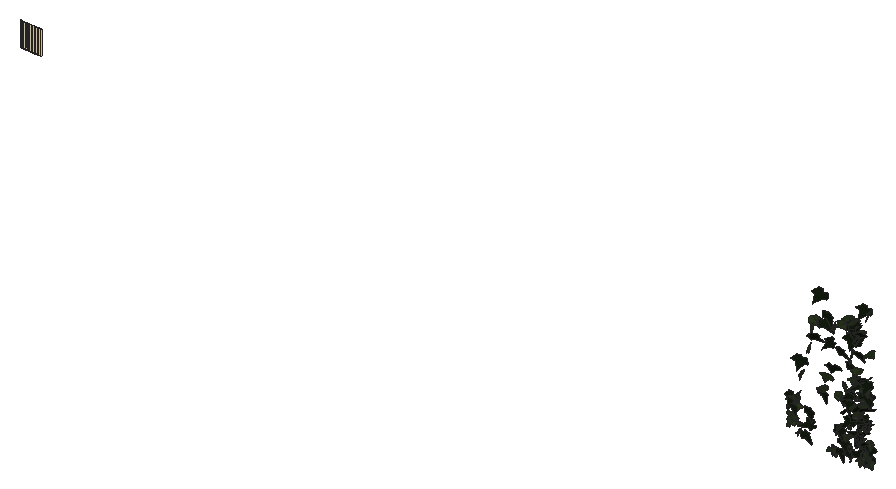
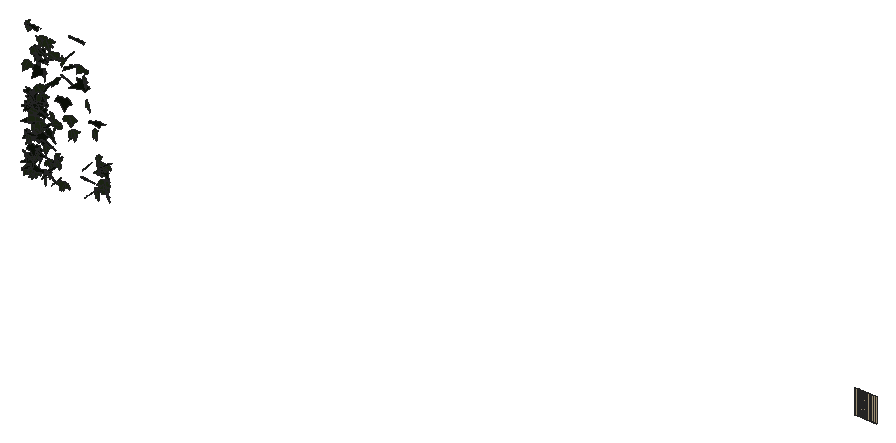
# SketchUp Ruby script. Lengths in inches.
U = 1.inch
M = Sketchup.active_model
def pt(a) = Geom::Point3d.new(a.map { |v| v * U })
def face(e, loops, mat)
  f = e.add_face(loops[0].map { |a| pt(a) })
  loops[1..].each { |l| e.add_face(l.map { |a| pt(a) }).erase! }
  f.material = f.back_material = mat if mat
  f
end
# faces: each face lists its corners as indices into pts; further lists are holes
def faces(e, pts, list, mat = nil) = list.each { |f| face(e, (f[0].is_a?(Array) ? f : [f]).map { |l| l.map { |i| pts[i] } }, mat) }
# xy, xz, yz: faces in a plane at the given z, y or x. An outline is a flat list of corners, or four numbers for a rectangle; further outlines are holes
def ring(l) = l.size == 4 ? [[l[0], l[1]], [l[2], l[1]], [l[2], l[3]], [l[0], l[3]]] : l.each_slice(2).to_a
def flat(e, list, mat, &to3) = list.each { |f| face(e, (f[0].is_a?(Array) ? f : [f]).map { |l| ring(l).map { |u, v| to3.(u, v) } }, mat) }
def xy(e, z, list, mat = nil) = flat(e, list, mat) { |x, y| [x, y, z] }
def xz(e, y, list, mat = nil) = flat(e, list, mat) { |x, z| [x, y, z] }
def yz(e, x, list, mat = nil) = flat(e, list, mat) { |y, z| [x, y, z] }
def lines(e, pts, list) = list.each { |a, b| e.add_line(pt(pts[a]), pt(pts[b])) }
# prism: a flat outline (further loops are holes) pulled along v
def prism(e, loops, v, mat = nil)
  f = face(e, loops, mat); d = Geom::Vector3d.new(v.map { |x| x * U })
  f.pushpull(f.normal.samedirection?(d) ? d.length : -d.length)
end
def box(e, o, s, mat = nil) = prism(e, [[o, [o[0] + s[0], o[1], o[2]], [o[0] + s[0], o[1] + s[1], o[2]], [o[0], o[1] + s[1], o[2]]]], [0, 0, s[2]], mat)
def at(x, y, z, deg = 0) = Geom::Transformation.translation(pt([x, y, z])) * Geom::Transformation.rotation(ORIGIN, Z_AXIS, deg.degrees)
def axes(o, x, y, z) = Geom::Transformation.new([*x, 0, *y, 0, *z, 0, *pt(o).to_a, 1])
def part(name) = M.definitions.add(name)
# library, detail: a bought-in or finely detailed component or shape, given as its bounding box
def library(name, o, s) = part(name).tap { |d| box(d.entities, o, s) }
def detail(e, o, s) = box(e.add_group.entities, o, s)
def put(e, d, t, mat = nil) = e.add_instance(d, t).tap { |i| i.material = mat if mat }
def group(e, t, mat = nil) = e.add_group.tap { |g| g.transformation = t; g.material = mat if mat }.entities
root = M.entities
M.materials.add("1026 AP 7946 SUNNY SIDE UP").color = [254, 231, 186]
M.materials.add("efeu1").color = [18, 25, 13]
M.materials.add("efeu2").color = [43, 57, 29]
c1 = part("ivyleaf_10")
p = [[0,0.5,-0.03],[-0.0625,2.02,-0.43],[-0.19,2.01,-0.46],[-0.54,1.05,-0.29],[-0.52,0.625,-0.18],[-0.83,0.76,-0.28],
  [-1.16,0.64,-0.33],[-1.15,0.33,-0.24],[-0.77,-0.39,0.02],[-0.3,-0.51,0.16],[0.04,-0.48,0.23],[-0.02,2.01,-0.4375],
  [-0.06,2.01,-0.43],[0.04,-0.49,0.23],[0.67,-0.49,0.14],[1.38,0.36,-0.2],[1.375,0.51,-0.24],[0.81,0.65,-0.19],
  [0.62,0.59,-0.15],[0.6,1.09,-0.28],[0.5,1.23,-0.31]]
faces(c1.entities,p,[[0,1,2,3,4,5,6,7,8,9,10],[11,12,0,13,14,15,16,17,18,19,20]],"efeu2")
c2 = part("ivyleaf_9")
p = [[1.54,2.16,1.25],[1.36,2.04,1.19],[-0.21,0.99,0.68],[-0.71,1.11,0.82],[-0.85,0.86,0.67],[-0.8,0.17,0.21],
  [-0.9,-0.01,0.1],[-0.67,-0.16,-0.02],[-0.08,-0.08,-0.05],[-0.03,-0.6,-0.4],[0.65,-0.88,-0.66],[0.83,-0.6,-0.49],
  [1.29,-0.42,-0.43],[1.8125,-0.07,-0.26],[1.21,0.44,0.15]]
faces(c2.entities,p,[[0,1,2,3,4,5,6,7,8,9,10,11,12,13,14]],"efeu1")
xz(root,213,[[29.49,274,29.64,276],[29.64,274,29.73,276],[29.73,274,29.74,276],[29.74,274,29.75,276]],"1026 AP 7946 SUNNY SIDE UP")
xz(root,213.01,[[29.18,274,29.21,276],[29.21,274,29.23,276],[29.23,274,29.37,276],[29.37,274,29.46,276],[29.46,274,29.47,276]],"1026 AP 7946 SUNNY SIDE UP")
xz(root,213.02,[[28.91,274,28.94,276],[28.94,274,28.98,276],[28.98,274,29.09,276]],"1026 AP 7946 SUNNY SIDE UP")
xz(root,213.03,[[28.68,274,28.72,276],[28.72,274,28.83,276]],"1026 AP 7946 SUNNY SIDE UP")
xz(root,213.04,[[28.5625,274,28.64,276]],"1026 AP 7946 SUNNY SIDE UP")
xz(root,213.05,[[28.37,274,28.42,276],[28.42,274,28.47,276]],"1026 AP 7946 SUNNY SIDE UP")
xz(root,213.07,[[28.03,274,28.1,276],[28.1,274,28.15,276]],"1026 AP 7946 SUNNY SIDE UP")
p = [[28.5625,213.04,276],[28.47,213.05,276],[28.47,213.05,274],[28.5625,213.04,274],[28.68,213.03,276],[28.64,213.04,276],
  [28.64,213.04,274],[28.68,213.03,274],[28.91,213.02,276],[28.83,213.03,276],[28.83,213.03,274],[28.91,213.02,274],
  [29.18,213.01,276],[29.09,213.02,276],[29.09,213.02,274],[29.18,213.01,274],[29.49,213,276],[29.47,213.01,276],
  [29.47,213.01,274],[29.49,213,274],[27.96,213.08,276],[27.89,213.09,276],[27.89,213.09,274],[27.96,213.08,274],
  [28.03,213.07,276],[28.03,213.07,274],[28.21,213.0625,276],[28.15,213.07,276],[28.15,213.07,274],[28.21,213.0625,274],
  [28.3,213.06,276],[28.3,213.06,274],[28.37,213.05,276],[28.37,213.05,274]]
faces(root,p,[[0,1,2,3],[4,5,6,7],[8,9,10,11],[12,13,14,15],[16,17,18,19],[20,21,22,23],[24,20,23,25],[26,27,28,29],
  [30,26,29,31],[32,30,31,33]],"1026 AP 7946 SUNNY SIDE UP")
put(root,c1,axes([92.42,213.08,268.59],[0.21828,-0.20306,-0.07657],[-0.06528,0.06026,-0.25305],[0.33305,0.14489,0.00059]),"1026 AP 7946 SUNNY SIDE UP")
put(root,c1,axes([92.74,212.95,269.25],[-0.4097,0.02552,0.01309],[-0.02552,-0.03834,-0.26681],[-0.03673,-0.25802,0.03938]),"1026 AP 7946 SUNNY SIDE UP")
put(root,c2,axes([92.6875,213.08,270.59],[-0.17756,-0.22686,0.08086],[-0.0304,-0.07928,-0.26092],[0.3769,-0.11327,0.01704]),"1026 AP 7946 SUNNY SIDE UP")
put(root,c1,axes([92.77,212.83,269.21],[-0.14311,0.23602,0.07022],[-0.10822,0.04384,-0.25584],[-0.37021,-0.10405,0.04764]),"1026 AP 7946 SUNNY SIDE UP")
put(root,c2,axes([92.93,212.8,270.07],[-0.1428,0.24975,-0.00668],[-0.00296,-0.00909,-0.27378],[-0.39289,-0.0907,0.00449]),"1026 AP 7946 SUNNY SIDE UP")
put(root,c1,axes([92.79,212.91,270.52],[-0.37063,-0.10251,-0.06698],[0.11383,-0.00629,-0.26256],[0.1526,-0.24427,0.03319]),"1026 AP 7946 SUNNY SIDE UP")
put(root,c1,axes([92.6,212.97,268.73],[0.00662,0.00721,0.26856],[0.3535,0.13195,-0.00673],[-0.20768,0.22482,-0.00289]),"1026 AP 7946 SUNNY SIDE UP")
put(root,c2,axes([92.84,212.91,270.16],[-0.00526,-0.26455,-0.04187],[-0.00961,0.03921,-0.27225],[0.4204,-0.00241,-0.00675]),"1026 AP 7946 SUNNY SIDE UP")
put(root,c1,axes([93,212.97,270.0625],[0.26463,0.20077,-0.04371],[-0.02853,-0.04158,-0.26982],[-0.32178,0.1688,-0.01202]),"1026 AP 7946 SUNNY SIDE UP")
put(root,c1,axes([93.21,213.04,270.48],[0.16765,-0.22108,-0.10492],[-0.02134,0.10426,-0.25027],[0.38132,0.10303,0.03213]),"1026 AP 7946 SUNNY SIDE UP")
put(root,c1,axes([93.23,212.99,270.95],[0.03829,-0.26848,0.00987],[0.00332,-0.01096,-0.27778],[0.4225,0.02442,0.00129]),"1026 AP 7946 SUNNY SIDE UP")
put(root,c1,axes([93.38,212.96,268.3125],[0.04559,-0.25312,0.02267],[-0.00043,-0.02362,-0.26259],[0.39971,0.02885,-0.00287]),"1026 AP 7946 SUNNY SIDE UP")
put(root,c2,axes([93.4375,213.06,273.625],[-0.33931,-0.1697,-0.05486],[0.08709,0.01386,-0.28175],[0.26529,-0.2216,0.02233]),"1026 AP 7946 SUNNY SIDE UP")
put(root,c1,axes([93.59,212.9375,272.71],[0.05303,-0.27391,0.0345],[0.0171,-0.03396,-0.28443],[0.43387,0.03482,0.007]),"1026 AP 7946 SUNNY SIDE UP")
put(root,c2,axes([93.7,212.99,268.1875],[0.13486,-0.22388,-0.09194],[-0.0002,0.09335,-0.24433],[0.37823,0.07988,0.03265]),"1026 AP 7946 SUNNY SIDE UP")
put(root,c1,axes([94.13,212.99,274.79],[-0.14037,0.25671,0.1001],[-0.24399,0.03558,-0.24722],[-0.35504,-0.12594,0.13032]),"1026 AP 7946 SUNNY SIDE UP")
put(root,c2,axes([94.38,213,269.03],[-0.37387,0.06985,0.08277],[-0.14776,-0.04725,-0.24567],[-0.07766,-0.24636,0.06898]),"1026 AP 7946 SUNNY SIDE UP")
put(root,c2,axes([94.08,212.99,270.03],[0.06407,-0.25983,0.03088],[-0.00633,-0.03245,-0.27098],[0.4115,0.03996,-0.00898]),"1026 AP 7946 SUNNY SIDE UP")
put(root,c1,axes([94.43,212.95,276.41],[0.21205,-0.26336,-0.02385],[0.00914,0.02726,-0.30411],[0.4154,0.13384,0.01887]),"1026 AP 7946 SUNNY SIDE UP")
put(root,c1,axes([94.57,212.9,277.12],[0.36582,0.06636,0.18243],[0.27242,0.03626,-0.2488],[-0.11782,0.2899,-0.00884]),"1026 AP 7946 SUNNY SIDE UP")
put(root,c2,axes([94.53,212.72,275.87],[0.40689,0.03962,0.1331],[0.20708,-0.01351,-0.26801],[-0.04613,0.28882,-0.02907]),"1026 AP 7946 SUNNY SIDE UP")
put(root,c2,axes([95.25,212.98,279.25],[-0.45392,-0.09147,-0.05492],[0.11094,-0.05269,-0.30371],[0.12358,-0.2887,0.07091]),"1026 AP 7946 SUNNY SIDE UP")
put(root,c1,axes([95.29,212.94,272.13],[-0.02515,-0.2748,-0.01568],[0.0061,0.01346,-0.28348],[0.43259,-0.01617,0.00308]),"1026 AP 7946 SUNNY SIDE UP")
put(root,c1,axes([95.36,212.99,272.15],[-0.2025,-0.23245,0.07228],[-0.00947,-0.07782,-0.27231],[0.38229,-0.12506,0.03154]),"1026 AP 7946 SUNNY SIDE UP")
put(root,c2,axes([95.27,212.97,271.85],[0.09402,-0.26054,0.05878],[0.01329,-0.05811,-0.27569],[0.41968,0.06021,-0.00444]),"1026 AP 7946 SUNNY SIDE UP")
put(root,c1,axes([95.625,213.01,273.13],[-0.41667,-0.0443,0.08007],[-0.11163,-0.04499,-0.27515],[0.08616,-0.27253,0.03073]),"1026 AP 7946 SUNNY SIDE UP")
put(root,c2,axes([95.35,213.03,277.15],[0.05543,-0.25001,-0.15925],[0.09631,0.15714,-0.2488],[0.45085,-0.00283,0.07273]),"1026 AP 7946 SUNNY SIDE UP")
put(root,c2,axes([95.64,212.98,277.76],[0.10916,-0.29078,0.0207],[-0.00111,-0.02252,-0.30805],[0.4585,0.06918,-0.00567]),"1026 AP 7946 SUNNY SIDE UP")
put(root,c2,axes([96.16,212.86,275.91],[-0.42304,0.06214,-0.05967],[0.08158,-0.03975,-0.27407],[-0.11698,-0.25243,0.02464]),"1026 AP 7946 SUNNY SIDE UP")
put(root,c1,axes([96.06,212.97,267.91],[-0.08072,0.23786,-0.08155],[0.00656,-0.08136,-0.25084],[-0.39481,-0.04998,0.0125]),"1026 AP 7946 SUNNY SIDE UP")
put(root,c2,axes([96.26,212.78,274.2],[0.30309,0.11804,-0.1485],[-0.17367,-0.09829,-0.22937],[-0.25821,0.20467,-0.02004]),"1026 AP 7946 SUNNY SIDE UP")
put(root,c1,axes([96.25,213.01,277.18],[-0.07571,0.09419,-0.26084],[-0.07709,-0.2474,-0.09648],[-0.43864,0.02722,0.06198]),"1026 AP 7946 SUNNY SIDE UP")
put(root,c1,axes([96.2,212.83,267.89],[-0.37314,-0.05397,-0.08215],[0.13704,-0.03207,-0.24596],[0.06344,-0.24819,0.0481]),"1026 AP 7946 SUNNY SIDE UP")
put(root,c1,axes([96.64,212.98,269.52],[0.00785,-0.26257,0.02857],[-0.01389,-0.02937,-0.27055],[0.41518,0.00398,-0.00959]),"1026 AP 7946 SUNNY SIDE UP")
put(root,c1,axes([96.74,212.97,269.79],[0.07961,-0.23788,0.1084],[0.02495,-0.10555,-0.25109],[0.4091,0.05273,-0.00578]),"1026 AP 7946 SUNNY SIDE UP")
put(root,c1,axes([97.03,213.07,277.44],[0.26109,0.01795,-0.22108],[-0.35017,-0.01488,-0.16588],[-0.03846,0.25725,0.00945]),"1026 AP 7946 SUNNY SIDE UP")
put(root,c2,axes([96.69,212.98,269.6],[0.00451,-0.26348,-0.02724],[0.00318,0.02497,-0.27129],[0.41614,0.00267,0.00237]),"1026 AP 7946 SUNNY SIDE UP")
put(root,c2,axes([96.73,212.96,267.93],[0.07791,-0.25125,0.02492],[0.00032,-0.02606,-0.26392],[0.39711,0.04932,-0.00468]),"1026 AP 7946 SUNNY SIDE UP")
put(root,c1,axes([96.875,212.9375,271.86],[-0.13635,0.22743,0.012],[-0.02312,0.00392,-0.25787],[-0.38564,-0.08065,0.01122]),"1026 AP 7946 SUNNY SIDE UP")
put(root,c2,axes([96.67,212.98,275.48],[0.28593,-0.22382,-0.03287],[0.03821,0.05848,-0.2912],[0.35315,0.17489,0.05812]),"1026 AP 7946 SUNNY SIDE UP")
put(root,c1,axes([96.65,212.78,272.11],[0.08298,0.03522,0.2574],[0.38153,0.08544,-0.06125],[-0.15477,0.22951,-0.01297]),"1026 AP 7946 SUNNY SIDE UP")
put(root,c1,axes([96.93,213.12,272.87],[-0.23462,0.15041,-0.13899],[0.09198,-0.12604,-0.2166],[-0.32677,-0.14347,0.03882]),"1026 AP 7946 SUNNY SIDE UP")
put(root,c2,axes([97.07,212.95,268.83],[-0.03593,-0.26132,0.01309],[0.00277,-0.0144,-0.2703],[0.41149,-0.02272,0.00296]),"1026 AP 7946 SUNNY SIDE UP")
put(root,c1,axes([97.31,212.97,269.22],[-0.25831,-0.16265,0.04576],[-0.02964,-0.04491,-0.23833],[0.28487,-0.15215,0.01669]),"1026 AP 7946 SUNNY SIDE UP")
put(root,c2,axes([97.55,212.77,271.39],[-0.16823,0.25064,-0.00533],[-0.00646,-0.00893,-0.2807],[-0.39419,-0.10682,0.00688]),"1026 AP 7946 SUNNY SIDE UP")
put(root,c2,axes([97.49,213,268.39],[-0.27483,0.11224,-0.10769],[0.11923,-0.07684,-0.21083],[-0.22825,-0.17528,0.01954]),"1026 AP 7946 SUNNY SIDE UP")
put(root,c1,axes([97.53,212.98,278.15],[-0.2204,-0.25983,0.06412],[0.00447,-0.07337,-0.30223],[0.42063,-0.13536,0.03681]),"1026 AP 7946 SUNNY SIDE UP")
put(root,c1,axes([97.45,212.99,268.37],[0.32536,-0.11446,0.01779],[0.01074,-0.0246,-0.23858],[0.19642,0.19094,-0.01641]),"1026 AP 7946 SUNNY SIDE UP")
put(root,c2,axes([97.74,212.93,270.54],[-0.4247,0.004,-0.02212],[0.03313,-0.02374,-0.27738],[-0.00921,-0.26991,0.02247]),"1026 AP 7946 SUNNY SIDE UP")
put(root,c2,axes([97.8,212.875,272.55],[-0.408,0.09704,-0.02415],[0.02454,-0.0266,-0.28485],[-0.15525,-0.25922,0.01845]),"1026 AP 7946 SUNNY SIDE UP")
put(root,c2,axes([97.73,212.9,267.95],[-0.16449,-0.20674,0.1211],[0.0624,0.11275,0.23893],[-0.36964,0.11103,-0.01356]),"1026 AP 7946 SUNNY SIDE UP")
put(root,c1,axes([97.64,212.96,270.22],[0.02068,-0.25768,-0.07879],[0.01136,0.07542,-0.26514],[0.42185,0.0106,0.011]),"1026 AP 7946 SUNNY SIDE UP")
put(root,c2,axes([97.53,212.97,271.85],[-0.0819,-0.26693,0.04277],[-0.00871,-0.04276,-0.28041],[0.42504,-0.05231,0.00249]),"1026 AP 7946 SUNNY SIDE UP")
put(root,c1,axes([97.78,212.91,267.88],[0.13614,-0.23728,-0.06479],[-0.00445,0.0643,-0.25911],[0.38542,0.08455,0.01989]),"1026 AP 7946 SUNNY SIDE UP")
put(root,c2,axes([97.57,212.97,274.61],[0.17894,-0.26311,0.0146],[-0.00229,-0.01769,-0.2953],[0.41444,0.1135,-0.00793]),"1026 AP 7946 SUNNY SIDE UP")
put(root,c1,axes([97.84,212.83,275.76],[0.1413,-0.25373,-0.12152],[0.00759,0.1238,-0.27316],[0.43896,0.07954,0.04384]),"1026 AP 7946 SUNNY SIDE UP")
put(root,c2,axes([97.79,212.99,276.76],[-0.21575,-0.26188,-0.01307],[0.01704,0.00696,-0.30447],[0.41181,-0.13749,0.00575]),"1026 AP 7946 SUNNY SIDE UP")
put(root,c2,axes([98.2,212.68,277.92],[-0.11183,0.17048,0.21124],[-0.28488,0.12528,-0.17612],[-0.33506,-0.16341,0.07924]),"1026 AP 7946 SUNNY SIDE UP")
put(root,c2,axes([97.72,212.94,277.48],[0.06843,-0.29164,0.05731],[0.00718,-0.05724,-0.30408],[0.46729,0.04359,-0.00372]),"1026 AP 7946 SUNNY SIDE UP")
put(root,c2,axes([98.19,213.03,277.46],[-0.28921,0.20601,0.01454],[-0.03322,-0.00207,-0.28569],[-0.34862,-0.1707,0.01516]),"1026 AP 7946 SUNNY SIDE UP")
put(root,c1,axes([98.08,212.91,273.84],[-0.19957,-0.25206,0.04744],[-0.0036,-0.05186,-0.29023],[0.40329,-0.12519,0.02089]),"1026 AP 7946 SUNNY SIDE UP")
put(root,c2,axes([97.79,212.83,272.67],[0.35821,-0.10644,0.06056],[0.07121,-0.04503,-0.25268],[0.19302,0.21415,-0.01917]),"1026 AP 7946 SUNNY SIDE UP")
put(root,c2,axes([98.21,212.88,270.94],[0.19363,0.12924,-0.21072],[-0.23247,-0.14254,-0.18465],[-0.30241,0.19233,0.00701]),"1026 AP 7946 SUNNY SIDE UP")
put(root,c2,axes([98.1875,212.9,268.83],[-0.05042,-0.13969,0.22872],[0.06846,0.21854,0.14888],[-0.4078,0.05396,-0.00328]),"1026 AP 7946 SUNNY SIDE UP")
put(root,c1,axes([98.08,212.76,278.15],[-0.22806,-0.2064,-0.10984],[0.11279,0.07579,-0.26221],[0.37257,-0.14929,0.01214]),"1026 AP 7946 SUNNY SIDE UP")
put(root,c1,axes([98.16,212.9375,271.76],[-0.1896,-0.24878,-0.02201],[0.01976,0.01608,-0.28468],[0.39194,-0.12116,0.0037]),"1026 AP 7946 SUNNY SIDE UP")
put(root,c2,axes([98.21,212.67,273.42],[0.09467,0.26452,0.08284],[-0.02161,0.08354,-0.27719],[-0.4335,0.0536,0.03191]),"1026 AP 7946 SUNNY SIDE UP")
put(root,c2,axes([98.47,212.89,269.58],[-0.19259,-0.01941,-0.24544],[-0.36638,-0.04946,0.12733],[-0.08306,0.26318,0.00743]),"1026 AP 7946 SUNNY SIDE UP")
put(root,c2,axes([98.27,213.16,273.37],[-0.34003,-0.11834,0.06904],[-0.07751,-0.05202,-0.24881],[0.2166,-0.2044,0.01935]),"1026 AP 7946 SUNNY SIDE UP")
put(root,c1,axes([98.27,212.95,274.48],[-0.18489,-0.2271,0.13318],[0.00266,-0.14377,-0.25689],[0.41189,-0.10101,0.06144]),"1026 AP 7946 SUNNY SIDE UP")
put(root,c2,axes([98.25,212.8,277.26],[0.33945,0.15846,-0.04362],[-0.03538,-0.04242,-0.27289],[-0.27638,0.20005,-0.01864]),"1026 AP 7946 SUNNY SIDE UP")
put(root,c2,axes([98.61,212.73,276.81],[-0.25924,0.18459,0.09705],[-0.13389,0.04849,-0.25404],[-0.32047,-0.16958,0.02763]),"1026 AP 7946 SUNNY SIDE UP")
put(root,c2,axes([98.32,212.95,273.79],[0.32743,0.17682,-0.08023],[-0.07968,-0.06204,-0.28142],[-0.29383,0.21386,-0.01309]),"1026 AP 7946 SUNNY SIDE UP")
put(root,c1,axes([98.26,212.64,271.17],[0.02844,-0.00361,0.26442],[0.03437,0.24679,0.00584],[-0.41799,0.02005,0.01847]),"1026 AP 7946 SUNNY SIDE UP")
put(root,c1,axes([98.38,212.96,276.875],[0.11289,-0.28823,0.00564],[-0.00058,-0.00742,-0.30604],[0.45336,0.07177,-0.00179]),"1026 AP 7946 SUNNY SIDE UP")
put(root,c2,axes([98.45,212.91,269.47],[-0.07081,-0.15364,0.22012],[0.07734,0.20895,0.166],[-0.40766,0.06633,-0.00674]),"1026 AP 7946 SUNNY SIDE UP")
put(root,c2,axes([98.24,212.85,275.82],[0.42075,-0.01933,-0.07409],[-0.11962,-0.0216,-0.265],[0.02165,0.25636,-0.02429]),"1026 AP 7946 SUNNY SIDE UP")
put(root,c1,axes([98.47,213.06,277.34],[-0.18032,-0.23035,0.07627],[0.00524,-0.08236,-0.27],[0.41081,-0.10006,0.03692]),"1026 AP 7946 SUNNY SIDE UP")
put(root,c2,axes([98.33,212.81,268.1],[-0.2437,0.03262,0.17494],[0.26921,-0.03759,0.15709],[0.08447,0.21392,0.00407]),"1026 AP 7946 SUNNY SIDE UP")
put(root,c1,axes([98.375,212.88,269.34],[-0.07544,0.25211,-0.07567],[0.01379,-0.07454,-0.26477],[-0.4133,-0.04851,0.00498]),"1026 AP 7946 SUNNY SIDE UP")
put(root,c2,axes([98.29,212.61,271.54],[0.06907,0.04754,0.26184],[0.3244,0.15207,-0.06372],[-0.26976,0.19505,-0.00959]),"1026 AP 7946 SUNNY SIDE UP")
put(root,c1,axes([98.43,212.9,269.41],[0.28508,-0.19273,0.04258],[0.02474,-0.04332,-0.27221],[0.30931,0.18109,-0.01748]),"1026 AP 7946 SUNNY SIDE UP")
put(root,c1,axes([98.49,213.01,269.28],[0.01024,0.21589,0.05569],[-0.02175,0.04948,-0.23005],[-0.37525,0.00302,0.01485]),"1026 AP 7946 SUNNY SIDE UP")
put(root,c2,axes([98.61,212.89,269.88],[0.13538,0.25087,-0.05063],[-0.00691,-0.0519,-0.27324],[-0.40234,0.0853,-0.01234]),"1026 AP 7946 SUNNY SIDE UP")
put(root,c2,axes([98.34,212.9,269.15],[0.23031,-0.22247,-0.00662],[0.01475,0.01235,-0.27391],[0.3496,0.14604,0.01592]),"1026 AP 7946 SUNNY SIDE UP")
put(root,c1,axes([98.68,212.85,271.98],[-0.38585,-0.1268,0.02064],[-0.0101,-0.03258,-0.28349],[0.20178,-0.2441,0.02528]),"1026 AP 7946 SUNNY SIDE UP")
put(root,c1,axes([98.81,212.93,272.57],[0.19184,0.03961,-0.21507],[-0.31411,-0.07986,-0.12908],[-0.15083,0.21669,-0.00472]),"1026 AP 7946 SUNNY SIDE UP")
put(root,c1,axes([98.68,212.9,271.47],[-0.02894,-0.27153,-0.04254],[-0.00495,0.04005,-0.28007],[0.43148,-0.01775,-0.00606]),"1026 AP 7946 SUNNY SIDE UP")
put(root,c2,axes([98.75,213.21,279.14],[-0.41521,-0.10106,-0.03879],[0.07828,-0.02104,-0.28088],[0.16377,-0.24618,0.0359]),"1026 AP 7946 SUNNY SIDE UP")
put(root,c2,axes([98.6875,212.6875,269.21],[0.19243,0.19814,-0.03385],[-0.01245,-0.03516,-0.24459],[-0.34109,0.11307,-0.01017]),"1026 AP 7946 SUNNY SIDE UP")
put(root,c2,axes([98.875,213.17,270.88],[-0.35969,-0.03163,0.06821],[-0.10047,-0.03496,-0.22831],[0.06811,-0.2186,0.02345]),"1026 AP 7946 SUNNY SIDE UP")
put(root,c1,axes([98.68,212.86,267.96],[-0.28397,-0.14049,-0.04886],[0.08017,0.01156,-0.23261],[0.2366,-0.17254,0.02018]),"1026 AP 7946 SUNNY SIDE UP")
put(root,c1,axes([98.6875,212.74,267.83],[-0.05012,-0.08743,-0.22691],[0.15648,0.18989,-0.09549],[0.35442,-0.0962,0.01007]),"1026 AP 7946 SUNNY SIDE UP")
put(root,c2,axes([98.7,213.01,268.7],[-0.02899,-0.006,-0.2415],[0.28082,-0.15408,-0.01118],[-0.26033,-0.16553,0.01483]),"1026 AP 7946 SUNNY SIDE UP")
put(root,c2,axes([98.95,212.89,273.9375],[0.00739,0.23532,0.053],[-0.04628,0.04663,-0.24959],[-0.40454,-0.00103,0.02952]),"1026 AP 7946 SUNNY SIDE UP")
put(root,c1,axes([99.09,212.8,267.84],[0.02344,-0.05002,-0.2525],[-0.25306,0.18307,-0.04849],[0.32028,0.14831,-0.01984]),"1026 AP 7946 SUNNY SIDE UP")
put(root,c2,axes([99.0625,212.875,270.8],[-0.36876,0.13455,-0.04954],[0.05004,-0.04242,-0.27798],[-0.21945,-0.23577,0.01986]),"1026 AP 7946 SUNNY SIDE UP")
put(root,c1,axes([98.86,212.72,268.46],[0.05583,0.22045,0.12083],[0.01076,0.11017,-0.23689],[-0.41807,0.03228,0.01004]),"1026 AP 7946 SUNNY SIDE UP")
put(root,c1,axes([99.04,212.81,270.5],[-0.08731,0.18163,0.14142],[-0.16915,0.10044,-0.19144],[-0.33904,-0.09688,0.05909]),"1026 AP 7946 SUNNY SIDE UP")
put(root,c2,axes([98.71,213.02,273.16],[0.17032,-0.18283,0.11803],[0.09631,-0.09733,-0.22461],[0.35157,0.11524,0.00435]),"1026 AP 7946 SUNNY SIDE UP")
put(root,c2,axes([98.74,212.73,271.74],[0.271,0.04266,0.18705],[0.23899,0.11459,-0.16661],[-0.18851,0.20661,0.05768]),"1026 AP 7946 SUNNY SIDE UP")
put(root,c2,axes([98.76,212.95,272.85],[-0.09684,-0.13324,-0.21027],[0.23319,0.14406,-0.14665],[0.32555,-0.14282,0.0425]),"1026 AP 7946 SUNNY SIDE UP")
put(root,c1,axes([98.9375,212.89,270.56],[-0.13116,-0.20099,-0.17146],[0.12025,0.14698,-0.22302],[0.39112,-0.11259,0.01107]),"1026 AP 7946 SUNNY SIDE UP")
put(root,c2,axes([99.03,212.9,268.89],[0.0837,0.15345,0.16178],[0.03463,0.14896,-0.16924],[-0.36156,0.04979,0.02124]),"1026 AP 7946 SUNNY SIDE UP")
put(root,c1,axes([98.8,212.87,273.28],[0.31222,0.03143,0.1582],[0.25345,-0.00664,-0.19807],[-0.03452,0.23559,-0.02334]),"1026 AP 7946 SUNNY SIDE UP")
put(root,c2,axes([99.07,212.93,273.8125],[-0.39025,-0.07112,-0.12783],[0.20384,-0.00878,-0.26284],[0.09369,-0.27716,0.0394]),"1026 AP 7946 SUNNY SIDE UP")
put(root,c1,axes([99.09,213.12,278.97],[0.11632,-0.19922,0.18399],[0.0859,-0.16703,-0.22781],[0.44124,0.08504,-0.00415]),"1026 AP 7946 SUNNY SIDE UP")
put(root,c2,axes([99,212.9,272.9],[-0.1393,-0.23287,-0.13891],[0.10644,0.11668,-0.25523],[0.40844,-0.10983,0.01914]),"1026 AP 7946 SUNNY SIDE UP")
put(root,c2,axes([99.22,213.1,268.17],[-0.18702,-0.15964,0.09821],[-0.06834,-0.08591,-0.2083],[0.30681,-0.11645,0.01347]),"1026 AP 7946 SUNNY SIDE UP")
put(root,c1,axes([99.18,212.96,276.03],[-0.17788,-0.2189,-0.16717],[0.12376,0.14056,-0.25297],[0.40898,-0.13774,0.00384]),"1026 AP 7946 SUNNY SIDE UP")
put(root,c2,axes([99.16,213.21,268.8125],[-0.12567,-0.19618,0.02204],[-0.00198,-0.02428,-0.22468],[0.33532,-0.07366,0.00694]),"1026 AP 7946 SUNNY SIDE UP")
put(root,c2,axes([99.17,212.72,270.48],[0.13127,0.09752,0.20926],[0.13624,0.17873,-0.12781],[-0.3428,0.10838,0.02933]),"1026 AP 7946 SUNNY SIDE UP")
put(root,c1,axes([99.19,212.9,268.43],[0.03877,0.20887,-0.05145],[-0.01398,-0.05018,-0.22563],[-0.36463,0.02413,0.00318]),"1026 AP 7946 SUNNY SIDE UP")
put(root,c1,axes([99.11,213.12,269.24],[0.2962,-0.07749,0.10674],[0.13967,-0.06148,-0.20411],[0.16439,0.19186,-0.01891]),"1026 AP 7946 SUNNY SIDE UP")
put(root,c1,axes([99.2,212.79,267.98],[-0.35935,-0.08539,-0.08372],[0.14133,-0.0023,-0.24206],[0.13476,-0.22527,0.03061]),"1026 AP 7946 SUNNY SIDE UP")
